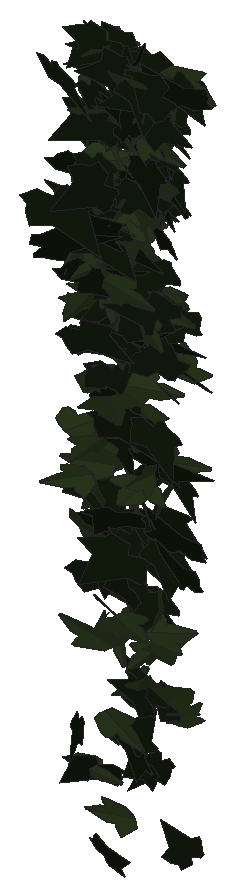
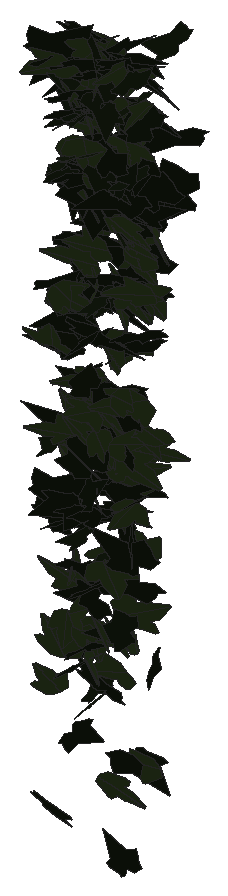
# SketchUp Ruby script. Lengths in millimetres.
U = 1.mm
M = Sketchup.active_model
def pt(a) = Geom::Point3d.new(a.map { |v| v * U })
def face(e, loops, mat)
  f = e.add_face(loops[0].map { |a| pt(a) })
  loops[1..].each { |l| e.add_face(l.map { |a| pt(a) }).erase! }
  f.material = f.back_material = mat if mat
  f
end
# faces: each face lists its corners as indices into pts; further lists are holes
def faces(e, pts, list, mat = nil) = list.each { |f| face(e, (f[0].is_a?(Array) ? f : [f]).map { |l| l.map { |i| pts[i] } }, mat) }
# xy, xz, yz: faces in a plane at the given z, y or x. An outline is a flat list of corners, or four numbers for a rectangle; further outlines are holes
def ring(l) = l.size == 4 ? [[l[0], l[1]], [l[2], l[1]], [l[2], l[3]], [l[0], l[3]]] : l.each_slice(2).to_a
def flat(e, list, mat, &to3) = list.each { |f| face(e, (f[0].is_a?(Array) ? f : [f]).map { |l| ring(l).map { |u, v| to3.(u, v) } }, mat) }
def xy(e, z, list, mat = nil) = flat(e, list, mat) { |x, y| [x, y, z] }
def xz(e, y, list, mat = nil) = flat(e, list, mat) { |x, z| [x, y, z] }
def yz(e, x, list, mat = nil) = flat(e, list, mat) { |y, z| [x, y, z] }
def lines(e, pts, list) = list.each { |a, b| e.add_line(pt(pts[a]), pt(pts[b])) }
# prism: a flat outline (further loops are holes) pulled along v
def prism(e, loops, v, mat = nil)
  f = face(e, loops, mat); d = Geom::Vector3d.new(v.map { |x| x * U })
  f.pushpull(f.normal.samedirection?(d) ? d.length : -d.length)
end
def box(e, o, s, mat = nil) = prism(e, [[o, [o[0] + s[0], o[1], o[2]], [o[0] + s[0], o[1] + s[1], o[2]], [o[0], o[1] + s[1], o[2]]]], [0, 0, s[2]], mat)
def at(x, y, z, deg = 0) = Geom::Transformation.translation(pt([x, y, z])) * Geom::Transformation.rotation(ORIGIN, Z_AXIS, deg.degrees)
def axes(o, x, y, z) = Geom::Transformation.new([*x, 0, *y, 0, *z, 0, *pt(o).to_a, 1])
def part(name) = M.definitions.add(name)
# library, detail: a bought-in or finely detailed component or shape, given as its bounding box
def library(name, o, s) = part(name).tap { |d| box(d.entities, o, s) }
def detail(e, o, s) = box(e.add_group.entities, o, s)
def put(e, d, t, mat = nil) = e.add_instance(d, t).tap { |i| i.material = mat if mat }
def group(e, t, mat = nil) = e.add_group.tap { |g| g.transformation = t; g.material = mat if mat }.entities
root = M.entities
M.materials.add("efeu1").color = [18, 25, 13]
M.materials.add("efeu2").color = [43, 57, 29]
c1 = part("ivyleaf_9")
p = [[39.1,54.8,31.7],[34.5,51.8,30.2],[-5.3,25.2,17.3],[-17.9,28.3,20.9],[-21.6,21.7,17],[-20.2,4.3,5.3],
  [-22.9,-0.3,2.5],[-17.1,-4,-0.6],[-2,-2.1,-1.2],[-0.7,-15.4,-10.1],[16.6,-22.3,-16.7],[21.1,-15.1,-12.5],
  [32.7,-10.7,-11],[46.1,-1.8,-6.6],[30.8,11.2,3.8]]
faces(c1.entities,p,[[0,1,2,3,4,5,6,7,8,9,10,11,12,13,14]],"efeu1")
c2 = part("ivyleaf_10")
p = [[0,12.8,-0.8],[-1.5,51.3,-10.9],[-4.9,51,-11.6],[-13.6,26.5,-7.3],[-13.2,15.9,-4.6],[-21.1,19.3,-7.2],
  [-29.5,16.3,-8.3],[-29.2,8.3,-6.2],[-19.7,-9.8,0.5],[-7.6,-13,4],[1,-12.2,5.8],[-0.4,51.1,-11.1],
  [-1.5,51.1,-10.9],[1,-12.4,5.9],[16.9,-12.4,3.5],[35.1,9.1,-5.1],[35,12.9,-6.1],[20.5,16.4,-4.9],
  [15.8,15,-3.8],[15.3,27.6,-7.1],[12.8,31.3,-7.8]]
faces(c2.entities,p,[[0,1,2,3,4,5,6,7,8,9,10],[11,12,0,13,14,15,16,17,18,19,20]],"efeu2")
put(root,c1,axes([2811.5,730.5,1493.9],[-1.89678,0.33655,-0.15122],[0.27024,-0.05215,-1.05191],[-0.64813,-1.00668,0.00394]))
put(root,c1,axes([2701.8,755.2,1420.9],[-0.04728,-0.85792,-0.79296],[0.27796,0.78464,-0.85349],[2.20597,-0.11726,0.09055]))
put(root,c1,axes([2676,765.7,1325.1],[0.74914,0.23601,1.0665],[1.74842,0.54173,-0.45895],[-1.12461,0.99945,-0.00309]))
put(root,c1,axes([2661.7,802.5,1613.8],[0.80896,-0.88524,0.22608],[0.20335,-0.19947,-0.98195],[1.72694,0.43817,0.00972]))
put(root,c1,axes([2703.1,809.5,488.7],[-0.10294,0.05349,-0.87386],[1.18919,-0.6109,-0.07607],[-1.16712,-0.62718,-0.00043]))
put(root,c2,axes([2776.7,807.1,1273.1],[-0.40491,0.09277,-0.83059],[1.44952,-0.33137,-0.2321],[-0.65492,-0.79078,-0.00018]))
put(root,c2,axes([2826.5,829.9,949.7],[-0.01216,0.02355,-0.9322],[-0.53948,-0.88815,-0.02049],[-1.69074,0.28322,0.01324]))
put(root,c1,axes([2706.6,814.3,1167.3],[0.04488,-0.21935,-0.82404],[0.51789,0.78319,-0.20069],[1.53808,-0.25731,0.09162]))
put(root,c1,axes([2718.9,827.8,1460.5],[0.16197,-0.8096,-0.26487],[-0.04404,0.26389,-0.81405],[1.6206,0.08809,0.00435]))
put(root,c2,axes([2755.7,820.6,1060.3],[-1.21031,-0.69411,-0.23654],[0.3056,0.17369,-0.94138],[1.36177,-0.65589,0.00103]))
put(root,c2,axes([2683.7,841.7,895.7],[0.42531,0.19537,-0.81594],[-1.2431,-0.48946,-0.29609],[-1.00222,0.69001,0.021]))
put(root,c1,axes([2696.5,847.1,1326.6],[-0.53582,-0.08244,0.94768],[1.10856,-0.79632,0.10377],[1.43136,0.58587,0.27439]))
put(root,c1,axes([2789.4,823,1536.8],[0.25213,0.21807,0.82631],[-0.1928,0.83429,-0.20394],[-1.61501,-0.06555,0.15335]))
put(root,c2,axes([2802.6,852.4,1193.1],[-0.46628,0.13324,-0.80396],[0.74902,-0.71577,-0.23856],[-1.35811,-0.4405,0.14446]))
put(root,c2,axes([2791.1,858.8,1538.8],[0.28098,-0.60488,0.75555],[0.45452,-0.71789,-0.62139],[1.78505,0.278,0.0393]))
put(root,c1,axes([2829.5,847.1,1603.1],[-1.79118,0.20242,0.21658],[-0.40498,0.04066,-0.96265],[-0.39284,-0.96488,0.00487]))
put(root,c2,axes([2761.2,836.7,674.6],[-1.08111,-0.47707,-0.52676],[0.819,0.30578,-0.74099],[1.07643,-0.7118,0.03473]))
put(root,c1,axes([2756.5,857.8,775.9],[-1.5717,-0.49425,0.21051],[-0.33298,-0.11756,-0.96236],[0.96668,-0.84408,0.01077]))
put(root,c1,axes([2793.7,859.1,1591.5],[-0.41243,-0.89598,0.17583],[-0.02921,-0.17711,-0.92144],[1.73751,-0.21565,0.02625]))
put(root,c1,axes([2834.6,857.2,1214],[-0.54853,-0.10694,0.83485],[-1.51131,-0.25797,-0.30719],[0.531,-0.84469,-0.01188]))
put(root,c1,axes([2767.6,864.7,442.4],[-0.07671,-0.66265,0.60596],[0.0389,-0.60709,-0.66252],[1.70851,-0.01593,0.04229]))
put(root,c2,axes([2655.1,857.1,1286.5],[0.90698,-0.76573,0.36457],[0.37194,-0.30778,-0.90191],[1.57065,0.51506,0.00305]))
put(root,c1,axes([2795.7,857.4,1463.7],[-0.90074,0.03178,-0.81915],[1.55275,-0.07392,-0.47424],[-0.15204,-0.94315,0.00957]))
put(root,c1,axes([2700.3,847.9,1322.6],[-0.40306,-0.51876,-0.81864],[0.7996,0.70598,-0.55606],[1.66219,-0.46541,0.06898]))
put(root,c2,axes([2732.1,853.4,486.2],[0.94581,-0.03874,0.73645],[1.40303,0.00195,-0.49736],[0.03817,0.88844,0.0332]))
put(root,c1,axes([2738.8,867.8,1599.5],[-0.55663,-0.1571,0.84291],[-1.05124,-0.64666,-0.31218],[1.24813,-0.61471,0.11298]))
put(root,c2,axes([2698.1,866,1259.8],[-0.05525,-0.37937,0.73832],[-0.1491,-0.73422,-0.38035],[1.57277,-0.08293,-0.01012]))
put(root,c1,axes([2713.7,859.2,1515.6],[-1.82748,-0.022,0.11467],[-0.21825,-0.00107,-0.96046],[0.04181,-0.96704,-0.00155]))
put(root,c1,axes([2728.6,866.9,1535.9],[0.47735,-0.78857,0.41667],[0.17572,-0.40755,-0.82689],[1.68832,0.26538,-0.03174]))
put(root,c2,axes([2762.6,851.9,1600],[-1.7338,0.12476,-0.14051],[0.26508,-0.01856,-0.91949],[-0.24005,-0.92158,-0.0005]))
put(root,c1,axes([2780.3,870,535.4],[0.29715,-0.8369,-0.20601],[0.18638,-0.19078,0.84925],[-1.62971,-0.17441,0.05956]))
put(root,c2,axes([2671.4,866.3,1190.5],[-0.41851,-0.7841,0.39939],[-0.17947,-0.3883,-0.81425],[1.66509,-0.23893,0.01262]))
put(root,c2,axes([2756.8,870.7,1375.6],[0.2378,0.40976,-0.73646],[-0.52535,-0.68354,-0.42715],[-1.5155,0.30125,0.03251]))
put(root,c1,axes([2751.1,860.8,1146.2],[-1.58746,0.23111,0.14881],[-0.26841,0.04828,-0.86548],[-0.44903,-0.84589,-0.00874]))
put(root,c1,axes([2778.2,875.9,416.3],[0.50259,-0.46942,-0.61497],[0.54814,-0.54346,0.5385],[-1.36659,-0.39062,-0.01017]))
put(root,c1,axes([2674.8,851.7,1225.5],[0.05879,-0.03752,1.01668],[1.93265,0.06315,-0.02852],[-0.11804,1.01518,0.03935]))
put(root,c2,axes([2780.8,863.7,903.7],[1.45692,0.14579,-0.33747],[-0.6327,-0.05824,-0.77925],[-0.29866,0.83456,0.00457]))
put(root,c1,axes([2801,869.4,1006],[0.08303,-0.95572,-0.15026],[-0.02214,0.14988,-0.95671],[1.84114,0.0449,-0.00473]))
put(root,c2,axes([2705.1,866.4,607.1],[-1.04289,-0.01997,-0.76744],[-1.4484,-0.1098,0.54625],[-0.19205,0.93657,0.04768]))
put(root,c2,axes([2685.1,859.1,1289.5],[-0.24013,-0.83042,-0.28085],[0.15825,0.27113,-0.83902],[1.66087,-0.1459,0.03934]))
put(root,c2,axes([2664.5,877,1492.9],[-0.22921,0.36573,-0.84418],[0.29947,-0.83065,-0.38231],[-1.72514,-0.19278,0.04579]))
put(root,c2,axes([2704.5,862.3,1249.4],[-1.14344,-0.09231,0.56672],[-1.07234,-0.06319,-0.60761],[0.21047,-0.82349,-0.0169]))
put(root,c2,axes([2728.1,862.7,1167.6],[0.17212,-1.00171,-0.21244],[-0.02973,0.21189,-1.00578],[1.94863,0.09171,0.00342]))
put(root,c2,axes([2707.9,865.2,1388.2],[-1.03403,-0.75573,0.04251],[-0.04753,-0.0344,-0.93076],[1.43979,-0.54389,-0.0002]))
put(root,c1,axes([2781.2,857.7,1389.6],[-1.6473,0.12266,0.31],[0.58292,-0.04806,0.87418],[0.2506,0.91812,0.00434]))
put(root,c2,axes([2703.9,869,1518.9],[-1.24727,-0.57392,0.21737],[-0.323,-0.13612,-0.87109],[1.12245,-0.67691,-0.00913]))
put(root,c1,axes([2731.6,866.4,836.3],[0.54672,0.56812,-0.5511],[-0.44557,-0.49905,-0.6365],[-1.43899,0.37038,-0.0123]))
put(root,c2,axes([2760.2,868,1309],[-1.12681,-0.6106,0.00529],[-0.00481,-0.00492,-0.85051],[1.16212,-0.59207,0.00161]))
put(root,c2,axes([2771,868.7,553.7],[-0.48015,-0.88779,-0.08894],[0.05364,0.08445,-0.92293],[1.69725,-0.25382,0.00401]))
put(root,c2,axes([2785.2,878,1592.5],[-0.2639,0.6043,-0.58634],[0.26139,-0.57005,-0.61999],[-1.58105,-0.19511,-0.00463]))
put(root,c1,axes([2736.5,885.1,703.7],[0.57901,-0.64303,-0.3925],[0.37592,-0.34041,0.71078],[-1.38363,-0.36158,0.02886]))
put(root,c1,axes([2759.6,864.7,451.2],[-0.96422,0.52755,0.4739],[0.60183,-0.35324,0.73129],[1.20804,0.59705,0.01393]))
put(root,c2,axes([2678.1,878.7,936.1],[-0.48403,-0.64363,0.4639],[-0.31731,-0.43291,-0.69205],[1.47625,-0.30408,0.00335]))
put(root,c2,axes([2707,879.6,1200.4],[1.12298,-0.40846,0.58896],[0.94675,-0.31582,-0.71741],[0.98206,0.77155,0.01814]))
put(root,c1,axes([2810.9,865.4,1115.3],[-1.34589,-0.19351,0.53672],[0.98834,0.13572,0.73315],[-0.44974,0.87735,0.00496]))
put(root,c1,axes([2808.3,860.7,1541.4],[0.5086,-0.26495,-0.76338],[-0.45836,0.74139,-0.34162],[1.468,0.32328,0.15781]))
put(root,c1,axes([2703.6,867.7,1313.9],[-0.06505,0.0148,-0.93069],[1.34172,0.60852,-0.01621],[1.15672,-0.70501,-0.03353]))
put(root,c2,axes([2679,876.6,852.4],[-1.38165,0.45602,0.20931],[0.32762,-0.11943,0.85725],[0.89699,0.74603,0.00929]))
put(root,c2,axes([2704.4,888.5,1482.1],[0.49304,-0.25932,0.86648],[1.15018,-0.62095,-0.36653],[1.28069,0.65751,-0.0044]))
put(root,c1,axes([2731.2,873,999.6],[-0.4606,-0.24807,-0.89384],[1.23454,0.61509,-0.34634],[1.26203,-0.69223,0.01258]))
put(root,c2,axes([2770.8,871.5,1376.3],[-1.46698,0.32663,0.14969],[-0.25835,0.0633,-0.83713],[-0.63312,-0.78264,-0.00523]))
put(root,c1,axes([2690.3,878.7,1335],[0.00376,0.04985,0.84064],[-1.56845,0.17301,-0.00832],[-0.32964,-0.82265,0.04919]))
put(root,c2,axes([2781.8,875.5,1213.4],[0.2382,0.04099,0.9297],[1.69677,0.26368,-0.13165],[-0.5078,0.90027,-0.00377]))
put(root,c2,axes([2801.6,886.8,1420.3],[-0.78202,-0.37972,0.66855],[-0.86968,-0.48901,-0.5586],[1.1768,-0.61372,0.03145]))
put(root,c2,axes([2653.9,886.1,1272],[-0.27628,-0.09052,-0.81757],[1.32447,-0.45612,-0.07307],[-0.83462,-0.69386,0.15469]))
put(root,c1,axes([2772.1,876.6,1169.6],[-1.6293,-0.23087,-0.17692],[-0.32572,-0.04484,0.88667],[-0.4476,0.87302,-0.00125]))
put(root,c1,axes([2779.2,896.5,1390.7],[0.18331,-0.66808,0.62784],[0.4017,-0.59818,-0.6689],[1.69799,0.21364,0.09046]))
put(root,c2,axes([2693,867,1431.8],[0.46538,0.18388,-0.87899],[1.24241,0.58919,0.30485],[1.17366,-0.69662,0.02583]))
put(root,c2,axes([2809.3,886.5,1397.2],[0.92498,-0.8469,0.10006],[0.08868,-0.08863,-0.97644],[1.62061,0.48823,-0.00368]))
put(root,c1,axes([2807.5,874.1,1352.1],[0.9526,-0.12141,-0.68792],[-1.2739,0.15881,-0.51503],[0.38043,0.83579,-0.00207]))
put(root,c1,axes([2669.7,885.8,1543.1],[0.70856,-0.80605,-0.21126],[-0.10038,0.20813,-0.88705],[1.58271,0.37406,0.03832]))
put(root,c1,axes([2833.3,889.4,1574.2],[0.94372,0.00518,0.83387],[-1.58143,0.08462,0.49359],[-0.1334,-0.96646,0.04768]))
put(root,c1,axes([2694.9,878.2,717.8],[0.73526,-0.48176,-0.56583],[-0.62435,0.46166,-0.61705],[1.26907,0.50624,0.02425]))
put(root,c1,axes([2644.8,893.8,1509.7],[0.92085,-0.67927,0.51897],[0.64463,-0.39519,-0.83304],[1.49376,0.58929,0.03957]))
put(root,c2,axes([2684.5,887.4,1192.8],[-1.15339,-0.43763,0.38033],[-0.59589,-0.21605,-0.74749],[0.92876,-0.68209,-0.00726]))
put(root,c1,axes([2661.3,881.9,1404.2],[0.84385,-0.66642,-0.42409],[-0.22836,0.42387,-0.79152],[1.48593,0.4436,0.1192]))
put(root,c2,axes([2637.2,880.2,948.5],[1.09566,0.06226,-0.5923],[1.10595,0.12173,0.5776],[0.24829,-0.81696,0.04092]))
put(root,c1,axes([2719,898.5,1180.9],[-1.1549,-0.40056,0.3226],[-0.53117,-0.16263,-0.72691],[0.82218,-0.66772,-0.01648]))
put(root,c2,axes([2761.2,885.4,1603.5],[-1.46252,0.12602,-0.35686],[0.6649,-0.0744,-0.77857],[-0.27699,-0.844,0.01534]))
put(root,c1,axes([2635.2,886.2,1383.7],[0.06109,-0.14683,0.97769],[1.79472,-0.28929,-0.07441],[0.56521,0.93447,0.13059]))
put(root,c1,axes([2772.1,896.9,1272],[-1.14222,-0.65943,-0.19569],[0.25409,0.1431,-0.89165],[1.28423,-0.61483,0.00236]))
put(root,c1,axes([2683.1,897.8,1625.7],[-1.40764,-0.3966,0.09658],[-0.17058,-0.03722,-0.83919],[0.7579,-0.74497,-0.00949]))
put(root,c1,axes([2675.8,890.8,371.1],[0.37329,0.36038,-0.73019],[-0.65313,-0.64453,-0.41029],[-1.40539,0.39526,-0.00328]))
put(root,c2,axes([2730.4,884.6,302.8],[0.58417,-0.14086,-0.77767],[-1.36027,0.30658,-0.33763],[0.64196,0.77781,-0.00775]))
put(root,c1,axes([2722.8,888.7,1602],[-1.44443,0.34085,0.31775],[-0.53316,0.15154,-0.83168],[-0.70871,-0.8087,-0.02193]))
put(root,c2,axes([2645.8,890,363],[-0.36002,0.06706,-0.77238],[1.43417,-0.17103,-0.1994],[-0.34693,-0.7766,-0.02279]))
put(root,c1,axes([2710.4,904.6,1426.1],[0.10156,-0.47697,0.67741],[0.36186,-0.65364,-0.47521],[1.53468,0.18569,0.06722]))
put(root,c2,axes([2790.4,891.3,640.9],[0.82351,-0.12005,-0.7589],[1.41868,-0.14557,0.44804],[-0.35452,-0.86138,0.03005]))
put(root,c1,axes([2808.5,893.2,1161.5],[-0.51736,0.74942,-0.55981],[0.25867,-0.54514,-0.79577],[-1.7614,-0.30018,0.04756]))
put(root,c2,axes([2679.8,905.1,887.5],[-0.2945,-0.11552,-0.93869],[-1.40042,-0.58286,0.19303],[-1.13082,0.7519,0.00542]))
put(root,c2,axes([2774.1,896.5,981.5],[-0.91526,-0.68642,0.26656],[-0.26302,-0.22858,-0.83794],[1.37653,-0.50007,0.01713]))
put(root,c1,axes([2783.1,891.5,516.8],[-0.90034,-0.69223,0.34621],[0.3756,0.28447,0.83843],[-1.42435,0.51258,0.00225]))
put(root,c1,axes([2677.1,899.8,857],[-0.7821,-0.81415,-0.4028],[0.44103,0.33351,-0.91051],[1.67156,-0.46893,0.05176]))
put(root,c1,axes([2699.4,884.3,779.4],[0.24154,0.04204,-0.83107],[-1.53865,0.20536,-0.11307],[0.37513,0.81524,0.07134]))
put(root,c1,axes([2651.6,887.5,1120.6],[0.42322,-0.48451,-0.67386],[-0.07192,0.691,-0.5093],[1.57795,0.16144,0.15752]))
put(root,c1,axes([2751,896.8,1360.8],[-1.37088,0.18837,0.3015],[-0.54291,0.10028,-0.74417],[-0.40377,-0.77439,-0.02303]))
put(root,c1,axes([2763.5,906,691.1],[-1.13426,-0.6159,-0.2281],[0.29855,0.16561,-0.85704],[1.2138,-0.61627,-0.00235]))
put(root,c2,axes([2682.5,894.8,1607.3],[-0.78978,-0.78058,-0.19292],[0.16537,0.1723,-0.88402],[1.52134,-0.42396,-0.00406]))
put(root,c1,axes([2696.4,902.8,1212.1],[-1.48169,0.07649,-0.13455],[0.25657,-0.0038,-0.78222],[-0.14468,-0.79006,-0.00927]))
put(root,c2,axes([2756.9,898.9,1338.8],[0.88937,0.11071,-0.69672],[-1.34261,0.07863,-0.46066],[0.00852,0.83523,0.13572]))
put(root,c2,axes([2761.4,889.7,1325.8],[-0.03902,0.8887,-0.32651],[-0.01361,0.32643,0.88893],[1.80186,0.02171,-0.00036]))
put(root,c2,axes([2798.3,885,687.6],[0.18861,-0.56246,-0.80506],[0.01472,0.80958,-0.56466],[1.86905,0.05038,0.08569]))
put(root,c1,axes([2770.9,901.2,916.8],[0.44293,-0.10442,0.87336],[1.45731,-0.4205,-0.25432],[0.82375,0.80006,-0.01968]))
put(root,c2,axes([2798.4,909,882.5],[0.4654,-0.81839,0.36845],[0.19949,-0.35323,-0.85414],[1.69645,0.26605,-0.00064]))
put(root,c2,axes([2747,899.8,1480.4],[0.50708,-0.01284,0.95425],[1.80027,0.13486,-0.2623],[-0.24072,0.98153,0.04852]))
put(root,c1,axes([2840.1,895.9,742.5],[0.38814,-0.26437,0.74015],[-0.74223,0.62985,0.33243],[-1.29868,-0.43899,0.03122]))
put(root,c2,axes([2634.5,909.1,754.5],[-0.92278,-0.00356,0.85233],[1.52071,-0.34323,0.4531],[0.56466,0.91855,0.17261]))
put(root,c2,axes([2686.3,909.9,905.2],[-0.93861,-0.46191,0.76436],[-0.98665,-0.56293,-0.67467],[1.38404,-0.71455,0.0374]))
put(root,c1,axes([2659.5,894.3,1452],[1.2375,0.02162,-0.51347],[-0.97425,-0.04616,-0.65018],[-0.0867,0.82723,-0.02286]))
put(root,c2,axes([2774.1,910.4,947.8],[-0.92216,0.0994,0.79103],[1.29499,-0.43086,0.47093],[0.79077,0.8215,0.15127]))
put(root,c1,axes([2777.1,894.7,1364.6],[-0.9681,-0.16923,0.60195],[1.14056,0.08952,0.53158],[-0.33965,0.78299,0.06932]))
put(root,c2,axes([2772.8,916.6,1182.5],[-0.32628,0.03539,0.8404],[0.42433,-0.82509,0.08023],[1.5436,0.23429,0.15558]))
put(root,c2,axes([2809,903.4,523.4],[-1.5407,-0.05323,0.43726],[0.83478,-0.01318,0.81044],[-0.07718,0.91998,0.03691]))
put(root,c1,axes([2733.8,901.4,782.1],[0.31249,-0.76771,-0.44035],[-0.06527,0.44201,-0.78339],[1.68314,0.15967,0.05138]))
put(root,c1,axes([2794.1,915.5,764.2],[-0.36145,-0.87616,0.1169],[-0.02368,-0.11691,-0.89642],[1.68211,-0.18991,0.0125]))
put(root,c1,axes([2724,915.2,1221.9],[-1.22296,-0.4605,0.26493],[-0.39132,-0.16781,-0.79039],[0.93231,-0.67449,0.01577]))
put(root,c2,axes([2698.9,906.4,960.6],[-0.7866,-0.01249,0.7715],[1.46672,-0.05002,0.41204],[0.07272,0.87381,0.03462]))
put(root,c1,axes([2704.7,909.7,1185.3],[0.7824,-0.79665,0.03566],[0.04363,-0.0283,-0.89643],[1.51708,0.41167,0.00739]))
put(root,c1,axes([2818.8,906.2,789.6],[0.96781,-0.35418,0.69409],[-1.03577,0.43175,0.61903],[-1.0614,-0.74427,0.0288]))
put(root,c2,axes([2761,905.1,1510.1],[0.42094,-0.82992,-0.15972],[-0.04878,0.15843,-0.85875],[1.60776,0.2221,0.01576]))
put(root,c2,axes([2759.9,917,1558.1],[0.13053,0.59315,-0.69627],[-0.23334,-0.68596,-0.59644],[-1.72508,0.13767,0.02799]))
put(root,c2,axes([2757,919.6,584.8],[-0.23427,-0.56005,0.66674],[-0.10056,-0.66732,-0.5703],[1.65415,-0.11989,0.05976]))
put(root,c1,axes([2706.6,918.8,1609.4],[-0.93725,-0.10914,0.68792],[-1.12149,-0.38391,-0.48275],[0.70679,-0.7539,0.14624]))
put(root,c1,axes([2751.4,889.2,1611.1],[-0.48259,0.2213,-0.84943],[-1.24923,0.53924,0.33642],[1.10919,0.7036,0.00933]))
put(root,c1,axes([2775.1,894.5,1518.3],[-0.14923,0.95808,0.01706],[-0.00957,-0.01753,0.96126],[1.82369,0.0783,0.00644]))
put(root,c1,axes([2668.7,912.1,1001.4],[0.27558,-0.08938,-0.85635],[1.63229,0.09143,0.13548],[0.14428,-0.86368,0.10296]))
put(root,c2,axes([2733,917.1,1207.5],[-0.26554,0.47632,-0.68271],[0.22971,-0.67334,-0.49445],[-1.56758,-0.17936,0.04319]))
put(root,c1,axes([2770.2,922.4,395.6],[-0.03654,0.00933,-0.83943],[0.54873,-0.7885,-0.01536],[-1.50052,-0.28858,0.01482]))
put(root,c1,axes([2673,925.2,829.3],[-0.51931,-0.58977,0.52273],[-0.32272,-0.49628,-0.64844],[1.46474,-0.31844,0.04246]))
put(root,c2,axes([2651.1,895.2,1543.4],[-0.01677,0.67359,0.56678],[-0.02669,0.56663,-0.67363],[-1.67522,-0.01577,0.00506]))
put(root,c2,axes([2689.1,917.8,591.4],[0.99422,-0.37085,0.59303],[0.93187,-0.33467,-0.6406],[0.9506,0.71594,0.00773]))
put(root,c1,axes([2646.8,915.7,1147.8],[-0.3922,-0.81278,-0.24845],[0.10362,0.2425,-0.83847],[1.61422,-0.21304,-0.00654]))
put(root,c1,axes([2801,923.1,903.9],[0.32231,-0.88776,0.31715],[0.10648,-0.31219,-0.90376],[1.791,0.17832,-0.00334]))
put(root,c2,axes([2686.3,919.3,1086.5],[-0.52803,0.16552,0.85045],[1.39186,-0.43407,0.32306],[0.88415,0.78218,-0.00068]))
put(root,c2,axes([2793.2,914.6,1539.2],[1.11308,-0.70705,0.10192],[0.13005,-0.07575,-0.91757],[1.35333,0.58881,0.00435]))
put(root,c1,axes([2826,909.1,1169.2],[-1.17836,-0.5843,0.22468],[0.31486,0.15205,0.85131],[-1.14906,0.64086,0.00287]))
put(root,c1,axes([2747.7,923.3,1516.3],[0.26557,-0.67261,0.56712],[0.61617,-0.49466,-0.66633],[1.55692,0.3105,0.16697]))
put(root,c1,axes([2735.9,911.3,1177],[-0.58858,0.43987,0.64221],[0.57626,-0.56864,0.53529],[1.3648,0.4298,0.05094]))
put(root,c1,axes([2794.2,925.3,1385.2],[0.86715,-0.7397,-0.20503],[0.21224,-0.17211,0.86875],[-1.44537,-0.46905,0.00456]))
put(root,c1,axes([2782,927.8,1588.8],[-1.21382,-0.50586,0.51395],[-0.6928,-0.36645,-0.8124],[1.18478,-0.73254,0.05149]))
put(root,c1,axes([2686.2,918.7,942.6],[-0.70021,-0.0118,-0.83624],[1.59165,0.00157,-0.36796],[0.01178,-0.91359,0.01016]))
put(root,c2,axes([2726.8,930.2,1411.4],[-0.08966,0.03685,0.93794],[0.05252,-0.93866,0.03827],[1.78569,0.02946,0.04597]))
put(root,c1,axes([2706.1,908.1,1478.7],[0.13651,-0.53209,-0.65439],[0.16598,0.65791,-0.52539],[1.59658,-0.0229,0.11057]))
put(root,c2,axes([2726.6,912.8,1273.8],[0.44917,-0.00578,0.78886],[1.48624,0.11838,-0.23277],[-0.21274,0.81485,0.03941]))
put(root,c2,axes([2652.6,919.4,588.5],[0.25926,-0.73977,-0.23015],[0.07442,-0.22682,0.7522],[-1.47262,-0.1417,-0.00251]))
put(root,c1,axes([2738.9,930.4,1587.6],[-1.07338,-0.36253,0.53342],[-0.68653,-0.41009,-0.66011],[1.01752,-0.65912,0.11732]))
put(root,c2,axes([2749.3,912.6,1330.4],[1.41067,-0.48035,0.11053],[-0.1628,0.07122,0.88315],[-0.92387,-0.74601,0.01315]))
put(root,c1,axes([2736.4,907.8,1365.9],[1.38563,0.41398,-0.46611],[-0.78544,-0.21707,-0.83741],[-0.88926,0.83678,0.01336]))
put(root,c1,axes([2648.3,932.6,1599.1],[-0.19038,-0.61858,0.60768],[0.24507,-0.61552,-0.60536],[1.63202,0.02027,0.16179]))
put(root,c1,axes([2662.7,926.3,193.6],[-0.07816,-0.1153,0.76827],[0.61622,-0.70188,-0.08803],[1.344,0.3151,0.08504]))
put(root,c2,axes([2719,927.9,833.3],[0.41498,-0.33188,0.65628],[0.85962,-0.47977,-0.39269],[1.10458,0.49806,0.05904]))
put(root,c2,axes([2663.7,919,1482.1],[1.59951,0.01766,0.03566],[0.06803,-0.00354,-0.84061],[-0.0333,0.84118,-0.00428]))
put(root,c1,axes([2764.5,906,1129.1],[1.16382,0.23935,0.46236],[0.8392,0.14114,-0.65624],[-0.52687,0.75352,-0.02394]))
put(root,c1,axes([2706.5,902,1315.4],[-0.03775,0.42959,0.71938],[-0.22354,0.71105,-0.42785],[-1.57892,-0.11094,0.04338]))
put(root,c2,axes([2670.2,931,1030.5],[-0.21154,-0.46317,0.65253],[-0.21677,-0.64293,-0.47576],[1.50744,-0.15745,0.02316]))
put(root,c2,axes([2665.1,909,827.6],[-0.68181,-0.52162,-0.58592],[0.65883,0.4729,-0.63266],[1.33977,-0.498,0.01293]))
put(root,c1,axes([2668.4,902.2,753.2],[-0.05667,-0.08491,0.96584],[0.4346,0.9385,0.08955],[-1.79337,0.23012,-0.00882]))
put(root,c2,axes([2741.1,911.4,1560.3],[-0.83056,0.67345,0.28048],[-0.37302,0.20659,-0.80097],[-1.33739,-0.47585,0.04922]))
put(root,c1,axes([2652.9,911.6,701],[0.11729,-0.34853,-0.91107],[0.75128,0.84371,-0.29606],[1.69769,-0.34929,0.19396]))
put(root,c1,axes([2787.2,931,498.4],[-0.06503,-0.74609,-0.23376],[0.07214,-0.23528,0.74543],[-1.48627,0.02123,0.04641]))
put(root,c1,axes([2749.4,928.4,1404.7],[-0.49519,-0.93373,-0.2218],[0.08766,0.2174,-0.9692],[1.82441,-0.26388,-0.01363]))
put(root,c2,axes([2736.3,927,533.2],[0.61156,-0.73321,0.24571],[0.18708,-0.22519,-0.80053],[1.45977,0.33603,-0.00034]))
put(root,c1,axes([2760.4,919.4,1511.9],[1.0997,-0.57472,-0.19355],[-0.21103,0.16271,-0.81417],[1.13472,0.58725,0.03616]))
put(root,c1,axes([2770.6,919.2,1402.1],[-0.99936,0.32717,0.51336],[-0.96331,0.14201,-0.60823],[-0.64369,-0.72048,0.11323]))
put(root,c1,axes([2783.7,936.1,1537],[-0.97055,-0.5231,0.43537],[-0.48442,-0.35796,-0.72823],[1.20127,-0.56698,0.05809]))
put(root,c1,axes([2800,919.6,1586.8],[-0.0764,-0.66698,-0.60192],[0.09722,0.59985,-0.66809],[1.70711,-0.06401,0.01111]))
put(root,c2,axes([2668.5,939,952.8],[-0.3247,-0.18924,0.88257],[0.07888,-0.89889,-0.18472],[1.71607,0.00551,0.17548]))
put(root,c1,axes([2771.8,932.7,1512.4],[-0.52632,-0.80923,-0.02822],[0.01687,0.02679,-0.85518],[1.54097,-0.27669,-0.00028]))
put(root,c1,axes([2752.8,918.3,818.6],[0.03662,-0.6235,0.67699],[-0.07143,0.67604,0.6237],[-1.75018,-0.04064,-0.01129]))
put(root,c1,axes([2681.6,922.6,1042.4],[-0.45739,-0.65657,-0.61162],[0.34512,0.58458,-0.69879],[1.67252,-0.30018,-0.02307]))
put(root,c2,axes([2652.5,916.3,1025.1],[-1.00439,-0.18632,-0.83131],[1.5229,0.22724,-0.55891],[0.55652,-0.95809,0.02911]))
put(root,c1,axes([2764.3,925.2,1098.3],[1.22205,-0.41493,0.35933],[0.60433,-0.17027,-0.76404],[0.8521,0.71583,0.02654]))
put(root,c1,axes([2646.3,937.1,1432.3],[0.08674,-0.79307,0.36204],[0.29853,-0.34916,-0.7846],[1.63213,0.10601,0.12427]))
put(root,c1,axes([2721.3,910,1533.5],[0.15843,0.80238,0.26686],[0.01033,0.26764,-0.80641],[-1.60929,0.08071,0.0211]))
put(root,c1,axes([2740.6,926.8,804.7],[-0.41665,-0.68621,-0.51465],[0.34679,0.48182,-0.71995],[1.59523,-0.28397,0.02209]))
put(root,c1,axes([2652.9,942.7,1422.1],[0.07664,-0.43997,0.81692],[0.18544,-0.81116,-0.44167],[1.75615,0.10486,0.01099]))
put(root,c1,axes([2756.7,925.6,1122.8],[-1.17617,0.23459,0.61311],[-1.10198,0.20199,-0.66091],[-0.58871,-0.84677,0.01221]))
put(root,c2,axes([2735.4,913.7,1037.8],[-0.25077,-0.2106,-0.90531],[1.39624,0.53787,-0.2319],[1.08619,-0.74003,0.08909]))
put(root,c1,axes([2747,944.5,1444.6],[-0.80877,-0.61016,0.47435],[0.04355,-0.55102,-0.68828],[1.47025,-0.31932,0.28132]))
put(root,c2,axes([2774.8,922.8,948.8],[0.89063,-0.31059,-0.62601],[-0.99473,0.34455,-0.56165],[0.88284,0.70154,-0.0013]))
put(root,c1,axes([2726.9,943.3,674.4],[-0.57681,-0.7837,0.34392],[-0.24084,-0.3198,-0.84026],[1.61093,-0.32842,-0.00248]))
put(root,c1,axes([2740.9,932.2,761.4],[0.73894,-0.6627,0.02723],[0.02593,-0.02357,-0.76806],[1.26204,0.3885,-0.00016]))
put(root,c2,axes([2782.7,917.1,923.2],[-0.06056,-0.00716,0.86582],[1.10755,0.64136,0.02669],[-1.22019,0.58251,-0.01874]))
put(root,c1,axes([2771.7,938.7,1422.9],[0.24847,-0.8422,0.12492],[0.03374,-0.12366,-0.85226],[1.62005,0.13175,-0.00141]))
put(root,c2,axes([2712,932.1,944.9],[-0.45331,-0.88275,0.12819],[-0.07297,-0.12243,-0.9143],[1.6961,-0.2412,-0.00507]))
put(root,c2,axes([2675.1,928.5,1343.4],[1.04377,-0.15889,-0.54624],[-1.01339,0.1237,-0.57059],[0.3811,0.7641,-0.02121]))
put(root,c1,axes([2636.4,934.9,748.7],[0.1883,-0.31834,0.81653],[1.31211,-0.47905,-0.2703],[1.02977,0.6686,0.19511]))
put(root,c2,axes([2749.3,945.7,625.3],[0.11216,-0.24243,0.86025],[0.5661,-0.80766,-0.24798],[1.60404,0.30199,0.02737]))
put(root,c1,axes([2767,929.5,901.6],[-1.22529,0.42685,-0.05787],[0.08909,-0.03413,-0.77245],[-0.81496,-0.6455,0.00257]))
put(root,c2,axes([2733,931.5,986.4],[-1.0334,0.17,-0.52108],[0.89079,-0.2379,-0.56533],[-0.54287,-0.71398,0.06429]))
put(root,c1,axes([2720.4,924.8,1127.3],[0.56202,-0.55151,-0.5727],[-0.29176,0.55997,-0.6183],[1.4848,0.31879,0.09528]))
put(root,c1,axes([2681.9,943.2,1445.1],[-0.39528,-0.1469,0.7938],[0.59779,-0.76977,-0.06027],[1.41535,0.28409,0.24715]))
put(root,c2,axes([2631.5,922.1,1228.2],[0.30003,0.17631,0.79245],[1.10157,0.54163,-0.23565],[-1.0834,0.59955,-0.02015]))
put(root,c1,axes([2652.6,935.1,621.4],[1.23764,-0.56004,0.19776],[0.28294,-0.13043,-0.85821],[1.09438,0.66707,-0.00177]))
put(root,c2,axes([2682.9,916.8,1610.5],[0.14781,-0.28098,-0.83386],[0.69175,0.77259,-0.22648],[1.52513,-0.32319,0.18354]))
put(root,c2,axes([2778.3,929.4,600.5],[-0.77525,-0.78012,-0.2349],[0.23284,0.20108,-0.87994],[1.53299,-0.42506,0.01486]))
put(root,c1,axes([2663,920,1394.5],[0.1682,-0.02853,-0.91244],[0.35224,0.89822,-0.01016],[1.70131,-0.18315,0.09231]))
put(root,c1,axes([2721.2,942.4,897.1],[1.58365,-0.20705,-0.28172],[0.53697,-0.03184,0.85674],[-0.39296,-0.87792,0.03537]))
put(root,c2,axes([2780.3,944.5,1184.2],[-0.4684,-0.34737,0.74132],[-0.8774,-0.58088,-0.42524],[1.28756,-0.52221,-0.0201]))
put(root,c1,axes([2740.3,934.1,1522.3],[0.64663,-0.66029,-0.33286],[-0.16411,0.32843,-0.73953],[1.39771,0.34404,0.06716]))
put(root,c1,axes([2710.6,938,1431.2],[-0.59214,0.5612,-0.46962],[0.19347,-0.47222,-0.63165],[-1.37921,-0.30718,0.11302]))
put(root,c2,axes([2793.5,926.2,1585.8],[0.8122,0.39564,0.752],[1.08578,0.49024,-0.58168],[-1.1985,0.71225,-0.01735]))
put(root,c2,axes([2694.3,936.9,719.5],[-1.27598,-0.47539,0.23155],[-0.35211,-0.13939,-0.82185],[0.94277,-0.69547,0.00644]))
put(root,c1,axes([2695,940,1203.9],[0.86404,-0.8519,-0.09464],[-0.08327,0.08393,-0.96532],[1.62918,0.4561,0.00085]))
put(root,c2,axes([2807.1,933.2,1081.1],[1.59593,-0.13043,0.06033],[-0.11311,0.01043,0.84864],[-0.24903,-0.84066,0.00117]))
put(root,c2,axes([2710.9,938,618.5],[0.9368,-0.71835,-0.05341],[-0.04577,0.04827,-0.87078],[1.37018,0.49276,0.00743]))
put(root,c1,axes([2713,937.7,661.4],[0.07946,0.00111,-0.78786],[1.43766,0.2241,0.04035],[0.42602,-0.75647,0.01079]))
put(root,c2,axes([2738.8,936.4,1461.5],[-1.37742,-0.41631,0.13122],[-0.20036,-0.0801,-0.83477],[0.80623,-0.73116,0.01674]))
put(root,c2,axes([2775.1,947.6,1193.6],[-0.54645,-0.7048,0.55914],[-0.20934,-0.55502,-0.7561],[1.69938,-0.29501,0.08666]))
put(root,c2,axes([2801.6,933.5,472.5],[-0.51013,-0.65007,0.30384],[0.23842,0.27697,0.7031],[-1.34471,0.29572,0.0094]))
put(root,c1,axes([2753.2,933,813.3],[-0.21934,-0.26802,-0.87115],[1.06072,0.67406,-0.28111],[1.37256,-0.56375,0.07803]))
put(root,c1,axes([2722.4,946.9,1041.6],[0.5038,-0.46113,0.55577],[0.55995,-0.47171,-0.53152],[1.25518,0.39553,0.01405]))
put(root,c1,axes([2824.5,928,250.7],[-1.17593,0.1312,-0.46593],[-0.86561,0.1012,0.63164],[0.31527,0.76721,-0.00364]))
